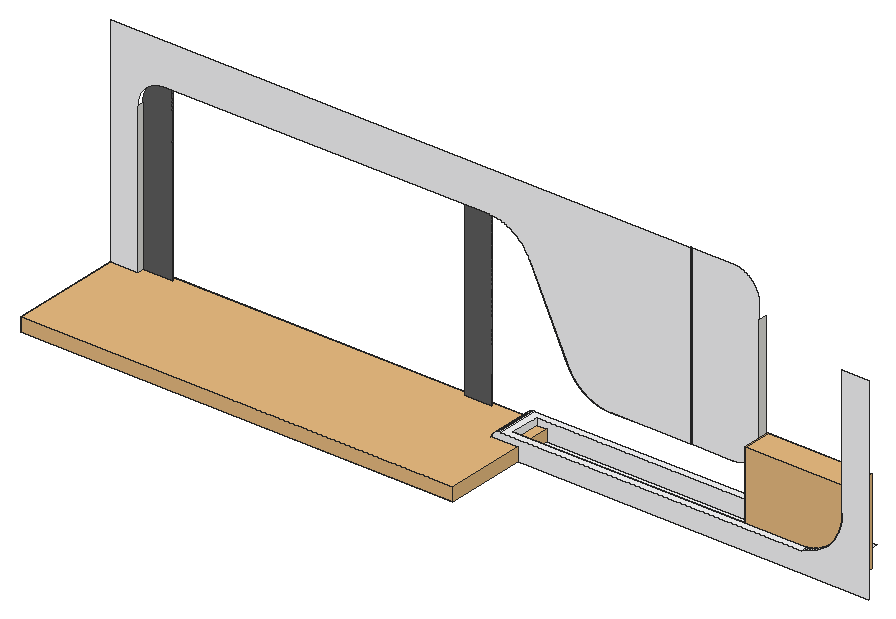
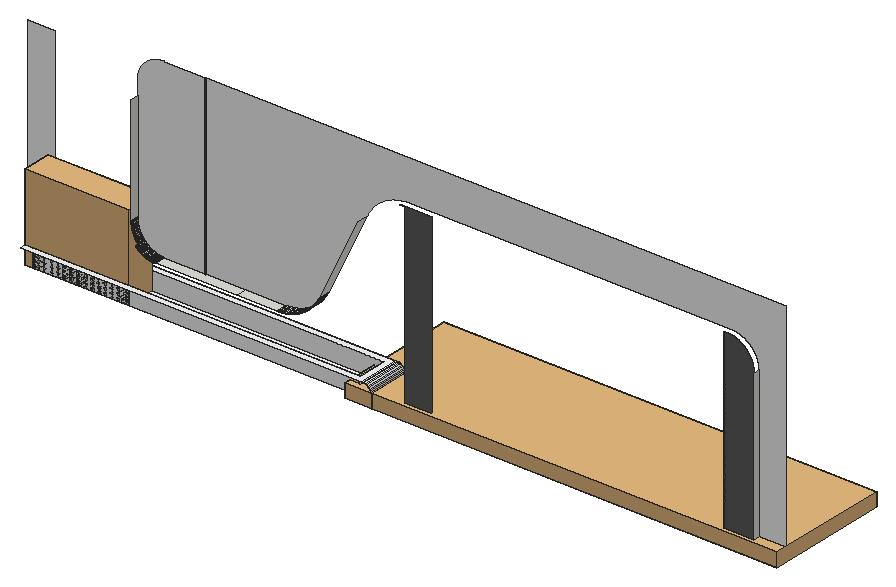
# SketchUp Ruby script. Lengths in inches.
U = 1.inch
M = Sketchup.active_model
def pt(a) = Geom::Point3d.new(a.map { |v| v * U })
def face(e, loops, mat)
  f = e.add_face(loops[0].map { |a| pt(a) })
  loops[1..].each { |l| e.add_face(l.map { |a| pt(a) }).erase! }
  f.material = f.back_material = mat if mat
  f
end
# faces: each face lists its corners as indices into pts; further lists are holes
def faces(e, pts, list, mat = nil) = list.each { |f| face(e, (f[0].is_a?(Array) ? f : [f]).map { |l| l.map { |i| pts[i] } }, mat) }
# xy, xz, yz: faces in a plane at the given z, y or x. An outline is a flat list of corners, or four numbers for a rectangle; further outlines are holes
def ring(l) = l.size == 4 ? [[l[0], l[1]], [l[2], l[1]], [l[2], l[3]], [l[0], l[3]]] : l.each_slice(2).to_a
def flat(e, list, mat, &to3) = list.each { |f| face(e, (f[0].is_a?(Array) ? f : [f]).map { |l| ring(l).map { |u, v| to3.(u, v) } }, mat) }
def xy(e, z, list, mat = nil) = flat(e, list, mat) { |x, y| [x, y, z] }
def xz(e, y, list, mat = nil) = flat(e, list, mat) { |x, z| [x, y, z] }
def yz(e, x, list, mat = nil) = flat(e, list, mat) { |y, z| [x, y, z] }
def lines(e, pts, list) = list.each { |a, b| e.add_line(pt(pts[a]), pt(pts[b])) }
# prism: a flat outline (further loops are holes) pulled along v
def prism(e, loops, v, mat = nil)
  f = face(e, loops, mat); d = Geom::Vector3d.new(v.map { |x| x * U })
  f.pushpull(f.normal.samedirection?(d) ? d.length : -d.length)
end
def box(e, o, s, mat = nil) = prism(e, [[o, [o[0] + s[0], o[1], o[2]], [o[0] + s[0], o[1] + s[1], o[2]], [o[0], o[1] + s[1], o[2]]]], [0, 0, s[2]], mat)
def at(x, y, z, deg = 0) = Geom::Transformation.translation(pt([x, y, z])) * Geom::Transformation.rotation(ORIGIN, Z_AXIS, deg.degrees)
def axes(o, x, y, z) = Geom::Transformation.new([*x, 0, *y, 0, *z, 0, *pt(o).to_a, 1])
def part(name) = M.definitions.add(name)
# library, detail: a bought-in or finely detailed component or shape, given as its bounding box
def library(name, o, s) = part(name).tap { |d| box(d.entities, o, s) }
def detail(e, o, s) = box(e.add_group.entities, o, s)
def put(e, d, t, mat = nil) = e.add_instance(d, t).tap { |i| i.material = mat if mat }
def group(e, t, mat = nil) = e.add_group.tap { |g| g.transformation = t; g.material = mat if mat }.entities
root = M.entities
M.materials.add("1421 AP 8232 ELEGANT GREY").color = [96, 96, 96]
M.materials.add("[Granite Tile]").color = [155, 148, 143]
M.materials.add("[Quartz Light Grey]").color = [251, 251, 252]
c1 = library("Group\#29",[0,-36,0],[192,55,6])
c2 = library("Mixed flower bed",[0,-29.95,0],[46.06,29.95,37.97])
xy(root,-17,[[187.5,39,333,52]],"[Quartz Light Grey]")
xy(root,-9,[[184.5,36,318,36,318,39,187.5,39,187.5,52,333,52,333,39,336,39,336,55,184.5,55]],"[Quartz Light Grey]")
xy(root,6,[[221.71,50,222,55],[222,50,240,55],[240,50,240,55,276,55,276,50,258,50,258,50.25,257.5,50.25,257.5,50],[276,50,276.16,55],[276.16,50,276.3125,55]])
xz(root,36,[[180,-18,348,-18,348,69,336,69,336,12,335.99,11.25,335.95,10.5,335.88,9.75,335.79,9,335.67,8.26,335.52,7.52,335.35,6.78,335.15,6.06,334.93,5.34,334.68,4.63,334.41,3.93,334.11,3.23,333.79,2.55,333.4375,1.89,333.07,1.23,332.68,0.59,332.26,-0.04,331.82,-0.65,331.36,-1.25,330.88,-1.83,330.38,-2.39,329.86,-2.9375,329.33,-3.46,328.77,-3.97,328.19,-4.46,327.6,-4.92,327,-5.37,326.37,-5.79,325.74,-6.19,325.08,-6.57,324.42,-6.92,323.74,-7.25,323.06,-7.56,322.36,-7.84,321.65,-8.1,320.93,-8.33,320.21,-8.54,319.48,-8.72,318.74,-8.87,318,-9,184.5,-9,183.91,-9.04,183.34,-9.15,182.78,-9.34,182.25,-9.6,181.76,-9.93,181.32,-10.32,180.93,-10.76,180.6,-11.25,180.34,-11.78,180.15,-12.34,180.04,-12.91,180,-13.5]],"[Quartz Light Grey]")
xz(root,39,[[187.5,-17,187.5,-9,318,-9,318.74,-8.87,319.48,-8.72,320.21,-8.54,320.93,-8.33,321.65,-8.1,322.36,-7.84,323.06,-7.56,323.74,-7.25,324.42,-6.92,325.08,-6.57,325.74,-6.19,326.37,-5.79,327,-5.37,327.6,-4.92,328.19,-4.46,328.77,-3.97,329.33,-3.46,329.86,-2.9375,330.38,-2.39,330.88,-1.83,331.36,-1.25,331.82,-0.65,332.26,-0.04,332.68,0.59,333.07,1.23,333.4375,1.89,333.79,2.55,334.11,3.23,334.41,3.93,334.68,4.63,334.93,5.34,335.15,6.06,335.35,6.78,335.52,7.52,335.67,8.26,335.79,9,335.88,9.75,335.95,10.5,335.99,11.25,336,12,336,-9,333,-9,333,-17]],"[Quartz Light Grey]")
xz(root,50,[[0,-18,12,-18,12,54.3125,12.01,54.47,12.02,54.63,12.03,54.78,12.05,55.1,12.07,55.25,12.08,55.41,12.1,55.57,12.125,55.72,12.15,55.88,12.17,56.03,12.2,56.1875,12.23,56.34,12.26,56.49,12.3,56.65,12.33,56.8,12.37,56.95,12.41,57.11,12.49,57.41,12.64,57.86,12.6875,58.01,12.74,58.15,12.8,58.3,12.85,58.45,12.91,58.59,12.97,58.74,13.04,58.88,13.1,59.02,13.17,59.17,13.45,59.73,13.53,59.86,13.61,60,13.6875,60.14,13.77,60.27,13.85,60.4,13.9375,60.54,14.02,60.67,14.2,60.93,14.29,61.05,14.38,61.18,14.48,61.31,14.58,61.43,14.67,61.55,14.77,61.67,14.98,61.91,15.08,62.03,15.1875,62.15,15.3,62.26,15.4,62.375,15.51,62.49,15.625,62.6,15.74,62.7,15.85,62.8125,15.97,62.92,16.09,63.02,16.33,63.23,16.45,63.33,16.57,63.42,16.69,63.52,16.82,63.62,16.95,63.71,17.07,63.8,17.33,63.98,17.46,64.0625,17.6,64.15,17.73,64.23,17.86,64.3125,18,64.39,18.14,64.47,18.27,64.55,18.83,64.83,18.98,64.9,19.12,64.96,19.26,65.03,19.41,65.09,19.55,65.15,19.7,65.2,19.85,65.26,19.99,65.3125,20.14,65.36,20.59,65.51,20.89,65.59,21.05,65.63,21.2,65.67,21.35,65.7,21.51,65.74,21.66,65.77,21.8125,65.8,21.97,65.83,22.12,65.85,22.28,65.875,22.43,65.9,22.59,65.92,22.75,65.93,22.9,65.95,23.22,65.97,23.37,65.98,23.53,65.99,23.6875,66,168.29,66,168.57,65.99,169.15,65.97,169.43,65.95,169.72,65.92,170,65.9,170.29,65.87,170.57,65.83,170.86,65.79,171.14,65.75,171.7,65.65,171.98,65.59,172.27,65.53,172.54,65.46,173.1,65.32,173.65,65.16,173.92,65.08,174.2,64.99,174.47,64.9,175.01,64.7,175.27,64.59,175.54,64.48,175.8,64.37,176.0625,64.25,176.32,64.13,176.58,64.01,176.84,63.88,177.09,63.75,177.35,63.61,177.6,63.48,177.84,63.33,178.09,63.1875,178.34,63.04,178.82,62.72,179.05,62.5625,179.29,62.4,179.52,62.23,179.75,62.0625,179.98,61.89,180.2,61.71,180.43,61.53,180.65,61.34,180.86,61.16,181.08,60.97,181.29,60.77,181.5,60.58,181.9,60.17,182.1,59.97,182.3,59.76,182.49,59.55,182.87,59.11,183.41,58.45,183.59,58.22,183.76,57.99,183.92,57.76,184.09,57.52,184.25,57.28,184.4,57.04,184.56,56.8,184.71,56.56,184.85,56.31,185,56.06,185.13,55.81,185.27,55.56,185.53,55.04,185.65,54.79,185.77,54.53,185.89,54.26,186,54,203.12,18,203.24,17.73,203.51,17.21,203.79,16.69,203.94,16.4375,204.09,16.18,204.25,15.93,204.4,15.68,204.5625,15.43,204.73,15.1875,204.9,14.95,205.24,14.47,205.42,14.23,205.78,13.77,205.97,13.54,206.16,13.32,206.36,13.1,206.55,12.875,206.75,12.66,206.96,12.45,207.16,12.23,207.37,12.03,207.58,11.82,208.24,11.22,208.68,10.84,208.91,10.65,209.14,10.47,209.38,10.29,209.61,10.11,210.09,9.77,210.34,9.6,210.58,9.44,210.83,9.28,211.33,8.97,211.59,8.82,211.84,8.68,212.1,8.53,212.36,8.39,212.89,8.13,213.15,8,213.96,7.64,214.23,7.53,214.51,7.42,214.78,7.32,215.0625,7.22,215.34,7.12,215.62,7.03,215.9,6.9375,216.18,6.85,216.47,6.77,216.75,6.69,217.04,6.62,217.32,6.55,217.9,6.43,218.1875,6.37,218.48,6.32,218.77,6.27,219.0625,6.22,219.35,6.18,219.65,6.14,219.9375,6.11,220.23,6.08,220.53,6.06,220.82,6.04,221.12,6.02,221.41,6.01,221.71,6,257.5,6,257.5,84,0,84],[258,6,276.3125,6,276.47,6.01,276.63,6.02,276.78,6.03,277.1,6.05,277.25,6.07,277.41,6.08,277.57,6.1,277.72,6.125,277.88,6.15,278.03,6.17,278.1875,6.2,278.34,6.23,278.49,6.26,278.65,6.3,278.8,6.33,278.95,6.37,279.11,6.41,279.41,6.49,279.86,6.64,280.01,6.6875,280.15,6.74,280.3,6.8,280.45,6.85,280.59,6.91,280.74,6.97,280.88,7.04,281.02,7.1,281.17,7.17,281.73,7.45,281.86,7.53,282,7.61,282.14,7.6875,282.27,7.77,282.4,7.85,282.54,7.9375,282.67,8.02,282.93,8.2,283.05,8.29,283.18,8.38,283.31,8.48,283.43,8.58,283.55,8.67,283.67,8.77,283.91,8.98,284.03,9.08,284.15,9.1875,284.26,9.3,284.375,9.4,284.49,9.51,284.6,9.625,284.7,9.74,284.8125,9.85,284.92,9.97,285.02,10.09,285.23,10.33,285.33,10.45,285.42,10.57,285.52,10.69,285.62,10.82,285.71,10.95,285.8,11.07,285.98,11.33,286.0625,11.46,286.15,11.6,286.23,11.73,286.3125,11.86,286.39,12,286.47,12.14,286.55,12.27,286.83,12.83,286.9,12.98,286.96,13.12,287.03,13.26,287.09,13.41,287.15,13.55,287.2,13.7,287.26,13.85,287.3125,13.99,287.36,14.14,287.51,14.59,287.59,14.89,287.63,15.05,287.67,15.2,287.7,15.35,287.74,15.51,287.77,15.66,287.8,15.8125,287.83,15.97,287.85,16.12,287.875,16.28,287.9,16.43,287.92,16.59,287.93,16.75,287.95,16.9,287.97,17.22,287.98,17.37,287.99,17.53,288,17.6875,288,72.3125,287.99,72.47,287.98,72.63,287.97,72.78,287.95,73.1,287.93,73.25,287.92,73.41,287.9,73.57,287.875,73.72,287.85,73.88,287.83,74.03,287.8,74.1875,287.77,74.34,287.74,74.49,287.7,74.65,287.67,74.8,287.63,74.95,287.59,75.11,287.51,75.41,287.36,75.86,287.3125,76.01,287.26,76.15,287.2,76.3,287.15,76.45,287.09,76.59,287.03,76.74,286.96,76.88,286.9,77.02,286.83,77.17,286.55,77.73,286.47,77.86,286.39,78,286.3125,78.14,286.23,78.27,286.15,78.4,286.0625,78.54,285.98,78.67,285.8,78.93,285.71,79.05,285.62,79.18,285.52,79.31,285.42,79.43,285.33,79.55,285.23,79.67,285.02,79.91,284.92,80.03,284.8125,80.15,284.7,80.26,284.6,80.375,284.49,80.49,284.375,80.6,284.26,80.7,284.15,80.8125,284.03,80.92,283.91,81.02,283.67,81.23,283.55,81.33,283.43,81.42,283.31,81.52,283.18,81.62,283.05,81.71,282.93,81.8,282.67,81.98,282.54,82.0625,282.4,82.15,282.27,82.23,282.14,82.3125,282,82.39,281.86,82.47,281.73,82.55,281.17,82.83,281.02,82.9,280.88,82.96,280.74,83.03,280.59,83.09,280.45,83.15,280.3,83.2,280.15,83.26,280.01,83.3125,279.86,83.36,279.41,83.51,279.11,83.59,278.95,83.63,278.8,83.67,278.65,83.7,278.49,83.74,278.34,83.77,278.1875,83.8,278.03,83.83,277.88,83.85,277.72,83.875,277.57,83.9,277.41,83.92,277.25,83.93,277.1,83.95,276.78,83.97,276.63,83.98,276.47,83.99,276.3125,84,258,84]],"[Quartz Light Grey]")
xz(root,50.25,[[257.5,6,258,84]])
xz(root,52,[[187.5,-17,333,-9]],"[Quartz Light Grey]")
xz(root,53,[[12,-18,25,-18,25,66,23.6875,66,23.53,65.99,23.37,65.98,23.22,65.97,22.9,65.95,22.75,65.93,22.59,65.92,22.43,65.9,22.28,65.875,22.12,65.85,21.97,65.83,21.8125,65.8,21.66,65.77,21.51,65.74,21.35,65.7,21.2,65.67,21.05,65.63,20.89,65.59,20.59,65.51,20.14,65.36,19.99,65.3125,19.85,65.26,19.7,65.2,19.55,65.15,19.41,65.09,19.26,65.03,19.12,64.96,18.98,64.9,18.83,64.83,18.27,64.55,18.14,64.47,18,64.39,17.86,64.3125,17.73,64.23,17.6,64.15,17.46,64.0625,17.33,63.98,17.07,63.8,16.95,63.71,16.82,63.62,16.69,63.52,16.57,63.42,16.45,63.33,16.33,63.23,16.09,63.02,15.97,62.92,15.85,62.8125,15.74,62.7,15.625,62.6,15.51,62.49,15.4,62.375,15.3,62.26,15.1875,62.15,15.08,62.03,14.98,61.91,14.77,61.67,14.67,61.55,14.58,61.43,14.48,61.31,14.38,61.18,14.29,61.05,14.2,60.93,14.02,60.67,13.9375,60.54,13.85,60.4,13.77,60.27,13.6875,60.14,13.61,60,13.53,59.86,13.45,59.73,13.17,59.17,13.1,59.02,13.04,58.88,12.97,58.74,12.91,58.59,12.85,58.45,12.8,58.3,12.74,58.15,12.6875,58.01,12.64,57.86,12.49,57.41,12.41,57.11,12.37,56.95,12.33,56.8,12.3,56.65,12.26,56.49,12.23,56.34,12.2,56.1875,12.17,56.03,12.15,55.88,12.125,55.72,12.1,55.57,12.08,55.41,12.07,55.25,12.05,55.1,12.03,54.78,12.02,54.63,12.01,54.47,12,54.3125],[25,-18,25.08,66],[155,-18,167,-18,167,65.97,169,65.97,168.86,65.98,168.57,65.99,168.29,66,155,66],[167,-18,167.08,65.97]],"1421 AP 8232 ELEGANT GREY")
yz(root,12,[[50,-18,53,54]])
yz(root,180,[[36,-18,55,-13.5]])
yz(root,187.5,[[39,-17,52,-9]],"[Quartz Light Grey]")
yz(root,257.5,[[50,6,50.25,84]])
yz(root,258,[[50,6,50.25,84]])
yz(root,288,[[50,17.6875,53.5,17.84],[50,17.84,53.5,18],[50,18,53.5,66]])
yz(root,333,[[39,-17,52,-9]])
p = [[180,36,-13.5],[180.04,36,-12.91],[180.04,55,-12.91],[180,55,-13.5],[180.15,36,-12.34],[180.15,55,-12.34],
  [180.34,36,-11.78],[180.34,55,-11.78],[180.6,36,-11.25],[180.6,55,-11.25],[180.93,36,-10.76],[180.93,55,-10.76],
  [181.32,36,-10.32],[181.32,55,-10.32],[181.76,36,-9.93],[181.76,55,-9.93],[182.25,36,-9.6],[182.25,55,-9.6],
  [182.78,36,-9.34],[182.78,55,-9.34],[183.34,36,-9.15],[183.34,55,-9.15],[183.91,36,-9.04],[183.91,55,-9.04],
  [184.5,36,-9],[184.5,55,-9],[318,36,-9],[318.74,36,-8.87],[318.74,39,-8.87],[318,39,-9],
  [319.48,36,-8.72],[319.48,39,-8.72],[320.21,36,-8.54],[320.21,39,-8.54],[320.93,36,-8.33],[320.93,39,-8.33],
  [321.65,36,-8.1],[321.65,39,-8.1],[322.36,36,-7.84],[322.36,39,-7.84],[323.06,36,-7.56],[323.06,39,-7.56],
  [323.74,36,-7.25],[323.74,39,-7.25],[324.42,36,-6.92],[324.42,39,-6.92],[325.08,36,-6.57],[325.08,39,-6.57],
  [325.74,36,-6.19],[325.74,39,-6.19],[326.37,36,-5.79],[326.37,39,-5.79],[327,36,-5.37],[327,39,-5.37],
  [327.6,36,-4.92],[327.6,39,-4.92],[328.19,36,-4.46],[328.19,39,-4.46],[328.77,36,-3.97],[328.77,39,-3.97],
  [329.33,36,-3.46],[329.33,39,-3.46],[329.86,36,-2.9375],[329.86,39,-2.9375],[330.38,36,-2.39],[330.38,39,-2.39],
  [330.88,36,-1.83],[330.88,39,-1.83],[331.36,36,-1.25],[331.36,39,-1.25],[331.82,36,-0.65],[331.82,39,-0.65],
  [332.26,36,-0.04],[332.26,39,-0.04],[332.68,36,0.59],[332.68,39,0.59],[333.07,36,1.23],[333.07,39,1.23],
  [333.4375,36,1.89],[333.4375,39,1.89],[333.79,36,2.55],[333.79,39,2.55],[334.11,36,3.23],[334.11,39,3.23],
  [334.41,36,3.93],[334.41,39,3.93],[334.68,36,4.63],[334.68,39,4.63],[334.93,36,5.34],[334.93,39,5.34],
  [335.15,36,6.06],[335.15,39,6.06],[220.53,55,6.06],[220.82,55,6.04],[220.82,50,6.04],[220.53,50,6.06],
  [221.12,55,6.02],[221.12,50,6.02],[221.41,55,6.01],[221.41,50,6.01],[221.71,55,6],[221.71,50,6],
  [276.3125,55,6],[276.47,55,6.01],[276.47,50,6.01],[276.3125,50,6],[276.63,55,6.02],[276.63,50,6.02],
  [276.78,55,6.03],[276.78,50,6.03],[276.94,55,6.04],[276.94,50,6.04],[277.1,55,6.05],[277.1,50,6.05],
  [335.35,36,6.78],[335.35,39,6.78],[219.35,55,6.18],[219.65,55,6.14],[219.65,50,6.14],[219.35,50,6.18],
  [219.9375,55,6.11],[219.9375,50,6.11],[220.23,55,6.08],[220.23,50,6.08],[277.25,55,6.07],[277.25,50,6.07],
  [277.41,55,6.08],[277.41,50,6.08],[277.57,55,6.1],[277.57,50,6.1],[277.72,55,6.125],[277.72,50,6.125],
  [277.88,55,6.15],[277.88,50,6.15],[278.03,55,6.17],[278.03,50,6.17],[218.77,55,6.27],[219.0625,55,6.22],
  [219.0625,50,6.22],[218.77,50,6.27],[278.1875,55,6.2],[278.1875,50,6.2],[278.34,55,6.23],[278.34,50,6.23],
  [278.49,55,6.26],[278.49,50,6.26],[218.1875,55,6.37],[218.48,55,6.32],[218.48,50,6.32],[218.1875,50,6.37],
  [278.65,55,6.3],[278.65,50,6.3],[278.8,55,6.33],[278.8,50,6.33],[278.95,55,6.37],[278.95,50,6.37],
  [217.61,55,6.49],[217.9,55,6.43],[217.9,50,6.43],[217.61,50,6.49],[279.11,55,6.41],[279.11,50,6.41],
  [279.26,55,6.45],[279.26,50,6.45],[217.32,55,6.55],[217.32,50,6.55],[279.41,55,6.49],[279.41,50,6.49],
  [279.56,55,6.54],[279.56,50,6.54],[279.71,55,6.59],[279.71,50,6.59],[216.75,55,6.69],[217.04,55,6.62],
  [217.04,50,6.62],[216.75,50,6.69],[279.86,55,6.64],[279.86,50,6.64],[280.01,55,6.6875],[280.01,50,6.6875],
  [216.47,55,6.77],[216.47,50,6.77],[280.15,55,6.74],[280.15,50,6.74],[280.3,55,6.8],[280.3,50,6.8],
  [335.52,36,7.52],[335.52,39,7.52],[216.18,55,6.85],[216.18,50,6.85],[280.45,55,6.85],[280.45,50,6.85],
  [215.62,55,7.03],[215.9,55,6.9375],[215.9,50,6.9375],[215.62,50,7.03],[280.59,55,6.91],[280.59,50,6.91],
  [280.74,55,6.97],[280.74,50,6.97],[215.34,55,7.12],[215.34,50,7.12],[280.88,55,7.04],[280.88,50,7.04],
  [281.02,55,7.1],[281.02,50,7.1],[215.0625,55,7.22],[215.0625,50,7.22],[281.17,55,7.17],[281.17,50,7.17],
  [214.78,55,7.32],[214.78,50,7.32],[281.31,55,7.24],[281.31,50,7.24],[281.45,55,7.31],[281.45,50,7.31],
  [214.51,55,7.42],[214.51,50,7.42],[281.59,55,7.38],[281.59,50,7.38],[214.23,55,7.53],[214.23,50,7.53],
  [281.73,55,7.45],[281.73,50,7.45],[335.67,36,8.26],[335.67,39,8.26],[213.96,55,7.64],[213.96,50,7.64],
  [281.86,55,7.53],[281.86,50,7.53],[282,55,7.61],[282,50,7.61],[213.69,55,7.76],[213.69,50,7.76],
  [282.14,55,7.6875],[282.14,50,7.6875],[282.27,55,7.77],[282.27,50,7.77],[213.42,55,7.88],[213.42,50,7.88],
  [282.4,55,7.85],[282.4,50,7.85],[213.15,55,8],[213.15,50,8],[282.54,55,7.9375],[282.54,50,7.9375],
  [282.67,55,8.02],[282.67,50,8.02],[212.89,55,8.13],[212.89,50,8.13],[282.8,55,8.11],[282.8,50,8.11],
  [212.625,55,8.26],[212.625,50,8.26],[282.93,55,8.2],[282.93,50,8.2],[283.05,55,8.29],[283.05,50,8.29],
  [335.79,36,9],[335.79,39,9],[212.36,55,8.39],[212.36,50,8.39],[283.18,55,8.38],[283.18,50,8.38],
  [212.1,55,8.53],[212.1,50,8.53],[283.31,55,8.48],[283.31,50,8.48],[211.84,55,8.68],[211.84,50,8.68],
  [283.43,55,8.58],[283.43,50,8.58],[283.55,55,8.67],[283.55,50,8.67],[211.59,55,8.82],[211.59,50,8.82],
  [283.67,55,8.77],[283.67,50,8.77],[211.33,55,8.97],[211.33,50,8.97],[283.79,55,8.875],[283.79,50,8.875],
  [283.91,55,8.98],[283.91,50,8.98],[335.88,36,9.75],[335.88,39,9.75],[211.08,55,9.125],[211.08,50,9.125],
  [284.03,55,9.08],[284.03,50,9.08],[210.83,55,9.28],[210.83,50,9.28],[284.15,55,9.1875],[284.15,50,9.1875],
  [284.26,55,9.3],[284.26,50,9.3],[210.58,55,9.44],[210.58,50,9.44],[284.375,55,9.4],[284.375,50,9.4],
  [210.34,55,9.6],[210.34,50,9.6],[284.49,55,9.51],[284.49,50,9.51],[284.6,55,9.625],[284.6,50,9.625],
  [210.09,55,9.77],[210.09,50,9.77],[284.7,55,9.74],[284.7,50,9.74],[335.95,36,10.5],[335.95,39,10.5],
  [284.8125,55,9.85],[284.8125,50,9.85],[209.85,55,9.94],[209.85,50,9.94],[209.61,55,10.11],[209.61,50,10.11],
  [284.92,55,9.97],[284.92,53.5,9.97],[284.92,50,9.97],[285.02,53.5,10.09],[285.02,50,10.09],[209.38,55,10.29],
  [209.38,50,10.29],[285.125,53.5,10.21],[285.125,50,10.21],[285.23,53.5,10.33],[285.23,50,10.33],[209.14,55,10.47],
  [209.14,50,10.47],[285.33,53.5,10.45],[285.33,50,10.45],[285.42,53.5,10.57],[285.42,50,10.57],[335.99,36,11.25],
  [335.99,39,11.25],[208.91,55,10.65],[208.91,50,10.65],[285.52,53.5,10.69],[285.52,50,10.69],[208.68,55,10.84],
  [208.68,50,10.84],[285.62,53.5,10.82],[285.62,50,10.82],[208.46,55,11.03],[208.46,50,11.03],[285.71,53.5,10.95],
  [285.71,50,10.95],[285.8,53.5,11.07],[285.8,50,11.07],[208.24,55,11.22],[208.24,50,11.22],[285.89,53.5,11.2],
  [285.89,50,11.2],[336,36,12],[336,39,12],[208.02,55,11.42],[208.02,50,11.42],[285.98,53.5,11.33],
  [285.98,50,11.33],[286.0625,53.5,11.46],[286.0625,50,11.46],[207.8,55,11.62],[207.8,50,11.62],[286.15,53.5,11.6],
  [286.15,50,11.6],[207.58,55,11.82],[207.58,50,11.82],[286.23,53.5,11.73],[286.23,50,11.73],[286.3125,53.5,11.86],
  [286.3125,50,11.86],[207.37,55,12.03],[207.37,50,12.03],[286.39,53.5,12],[286.39,50,12],[207.16,55,12.23],
  [207.16,50,12.23],[286.47,53.5,12.14],[286.47,50,12.14],[286.55,53.5,12.27],[286.55,50,12.27],[206.96,55,12.45],
  [206.96,50,12.45],[286.62,53.5,12.41],[286.62,50,12.41],[206.75,55,12.66],[206.75,50,12.66],[286.69,53.5,12.55],
  [286.69,50,12.55],[286.76,53.5,12.69],[286.76,50,12.69],[206.55,55,12.875],[206.55,50,12.875],[286.83,53.5,12.83],
  [286.83,50,12.83],[286.9,53.5,12.98],[286.9,50,12.98],[206.36,55,13.1],[206.36,50,13.1],[286.96,53.5,13.12],
  [286.96,50,13.12],[206.16,55,13.32],[206.16,50,13.32],[287.03,53.5,13.26],[287.03,50,13.26],[205.97,55,13.54],
  [205.97,50,13.54],[287.09,53.5,13.41],[287.09,50,13.41],[287.15,53.5,13.55],[287.15,50,13.55],[205.78,55,13.77],
  [205.78,50,13.77],[287.2,53.5,13.7],[287.2,50,13.7],[287.26,53.5,13.85],[287.26,50,13.85],[205.6,55,14],
  [205.6,50,14],[287.3125,53.5,13.99],[287.3125,50,13.99],[205.42,55,14.23],[205.42,50,14.23],[287.36,53.5,14.14],
  [287.36,50,14.14],[287.41,53.5,14.29],[287.41,50,14.29],[205.24,55,14.47],[205.24,50,14.47],[287.46,53.5,14.44],
  [287.46,50,14.44],[287.51,53.5,14.59],[287.51,50,14.59],[205.07,55,14.71],[205.07,50,14.71],[287.55,53.5,14.74],
  [287.55,50,14.74],[204.9,55,14.95],[204.9,50,14.95],[287.59,53.5,14.89],[287.59,50,14.89],[204.73,55,15.1875],
  [204.73,50,15.1875],[287.63,53.5,15.05],[287.63,50,15.05],[287.67,53.5,15.2],[287.67,50,15.2],[204.5625,55,15.43],
  [204.5625,50,15.43],[287.7,53.5,15.35],[287.7,50,15.35],[204.4,55,15.68],[204.4,50,15.68],[287.74,53.5,15.51],
  [287.74,50,15.51],[287.77,53.5,15.66],[287.77,50,15.66],[204.25,55,15.93],[204.25,50,15.93],[287.8,53.5,15.8125],
  [287.8,50,15.8125],[287.83,53.5,15.97],[287.83,50,15.97],[204.09,55,16.18],[204.09,50,16.18],[287.85,53.5,16.12],
  [287.85,50,16.12],[287.875,53.5,16.28],[287.875,50,16.28],[203.94,55,16.4375],[203.94,50,16.4375],[287.9,53.5,16.43],
  [287.9,50,16.43],[203.79,55,16.69],[203.79,50,16.69],[287.92,53.5,16.59],[287.92,50,16.59],[287.93,53.5,16.75],
  [287.93,50,16.75],[203.65,55,16.95],[203.65,50,16.95],[287.95,53.5,16.9],[287.95,50,16.9],[203.51,55,17.21],
  [203.51,50,17.21],[287.96,53.5,17.06],[287.96,50,17.06],[287.97,53.5,17.22],[287.97,50,17.22],[203.375,55,17.47],
  [203.375,50,17.47],[287.98,53.5,17.37],[287.98,50,17.37],[287.99,53.5,17.53],[287.99,50,17.53],[203.24,55,17.73],
  [203.24,50,17.73],[288,53.5,17.6875],[288,50,17.6875],[203.12,55,18],[203.12,50,18],[186,55,54],
  [186,50,54]]
faces(root,p,[[0,1,2,3],[1,4,5,2],[4,6,7,5],[6,8,9,7],[8,10,11,9],[10,12,13,11],[12,14,15,13],[14,16,17,15],
  [16,18,19,17],[18,20,21,19],[20,22,23,21],[22,24,25,23]],"[Quartz Light Grey]")
faces(root,p,[[26,27,28,29],[27,30,31,28],[30,32,33,31],[32,34,35,33],[34,36,37,35],[36,38,39,37],[38,40,41,39],[40,42,43,41],
  [42,44,45,43],[44,46,47,45],[46,48,49,47],[48,50,51,49],[50,52,53,51],[52,54,55,53],[54,56,57,55],[56,58,59,57],
  [58,60,61,59],[60,62,63,61],[62,64,65,63],[64,66,67,65],[66,68,69,67],[68,70,71,69],[70,72,73,71],[72,74,75,73],
  [74,76,77,75],[76,78,79,77],[78,80,81,79],[80,82,83,81],[82,84,85,83],[84,86,87,85],[86,88,89,87],[88,90,91,89],
  [92,93,94,95],[93,96,97,94],[96,98,99,97],[98,100,101,99],[102,103,104,105],[103,106,107,104],[106,108,109,107],[108,110,111,109],
  [110,112,113,111],[90,114,115,91],[116,117,118,119],[117,120,121,118],[120,122,123,121],[122,92,95,123],[112,124,125,113],[124,126,127,125],
  [126,128,129,127],[128,130,131,129],[130,132,133,131],[132,134,135,133],[136,137,138,139],[137,116,119,138],[134,140,141,135],[140,142,143,141],
  [142,144,145,143],[146,147,148,149],[147,136,139,148],[144,150,151,145],[150,152,153,151],[152,154,155,153],[156,157,158,159],[157,146,149,158],
  [154,160,161,155],[160,162,163,161],[164,156,159,165],[162,166,167,163],[166,168,169,167],[168,170,171,169],[172,173,174,175],[173,164,165,174],
  [170,176,177,171],[176,178,179,177],[180,172,175,181],[178,182,183,179],[182,184,185,183],[114,186,187,115],[188,180,181,189],[184,190,191,185],
  [192,193,194,195],[193,188,189,194],[190,196,197,191],[196,198,199,197],[200,192,195,201],[198,202,203,199],[202,204,205,203],[206,200,201,207],
  [204,208,209,205],[210,206,207,211],[208,212,213,209],[212,214,215,213],[216,210,211,217],[214,218,219,215],[220,216,217,221],[218,222,223,219],
  [186,224,225,187],[226,220,221,227],[222,228,229,223],[228,230,231,229],[232,226,227,233],[230,234,235,231],[234,236,237,235],[238,232,233,239],
  [236,240,241,237],[242,238,239,243],[240,244,245,241],[244,246,247,245],[248,242,243,249],[246,250,251,247],[252,248,249,253],[250,254,255,251],
  [254,256,257,255],[224,258,259,225],[260,252,253,261],[256,262,263,257],[264,260,261,265],[262,266,267,263],[268,264,265,269],[266,270,271,267],
  [270,272,273,271],[274,268,269,275],[272,276,277,273],[278,274,275,279],[276,280,281,277],[280,282,283,281],[258,284,285,259],[286,278,279,287],
  [282,288,289,283],[290,286,287,291],[288,292,293,289],[292,294,295,293],[296,290,291,297],[294,298,299,295],[300,296,297,301],[298,302,303,299],
  [302,304,305,303],[306,300,301,307],[304,308,309,305],[284,310,311,285],[308,312,313,309],[314,306,307,315],[316,314,315,317],[312,318,319,320,313],
  [320,319,321,322],[323,316,317,324],[322,321,325,326],[326,325,327,328],[329,323,324,330],[328,327,331,332],[332,331,333,334],[310,335,336,311],
  [337,329,330,338],[334,333,339,340],[341,337,338,342],[340,339,343,344],[345,341,342,346],[344,343,347,348],[348,347,349,350],[351,345,346,352],
  [350,349,353,354],[335,355,356,336],[357,351,352,358],[354,353,359,360],[360,359,361,362],[363,357,358,364],[362,361,365,366],[367,363,364,368],
  [366,365,369,370],[370,369,371,372],[373,367,368,374],[372,371,375,376],[377,373,374,378],[376,375,379,380],[380,379,381,382],[383,377,378,384],
  [382,381,385,386],[387,383,384,388],[386,385,389,390],[390,389,391,392],[393,387,388,394],[392,391,395,396],[396,395,397,398],[399,393,394,400],
  [398,397,401,402],[403,399,400,404],[402,401,405,406],[407,403,404,408],[406,405,409,410],[410,409,411,412],[413,407,408,414],[412,411,415,416],
  [416,415,417,418],[419,413,414,420],[418,417,421,422],[423,419,420,424],[422,421,425,426],[426,425,427,428],[429,423,424,430],[428,427,431,432],
  [432,431,433,434],[435,429,430,436],[434,433,437,438],[439,435,436,440],[438,437,441,442],[443,439,440,444],[442,441,445,446],[446,445,447,448],
  [449,443,444,450],[448,447,451,452],[453,449,450,454],[452,451,455,456],[456,455,457,458],[459,453,454,460],[458,457,461,462],[462,461,463,464],
  [465,459,460,466],[464,463,467,468],[468,467,469,470],[471,465,466,472],[470,469,473,474],[475,471,472,476],[474,473,477,478],[478,477,479,480],
  [481,475,476,482],[480,479,483,484],[485,481,482,486],[484,483,487,488],[488,487,489,490],[491,485,486,492],[490,489,493,494],[494,493,495,496],
  [497,491,492,498],[496,495,499,500],[501,497,498,502],[503,501,502,504]])
put(root,c1,at(0,36,-18),"[Granite Tile]")
put(root,c2,axes([290.43,52,-17],[1,0,0],[0,0.43409,0],[0,0,1]))
